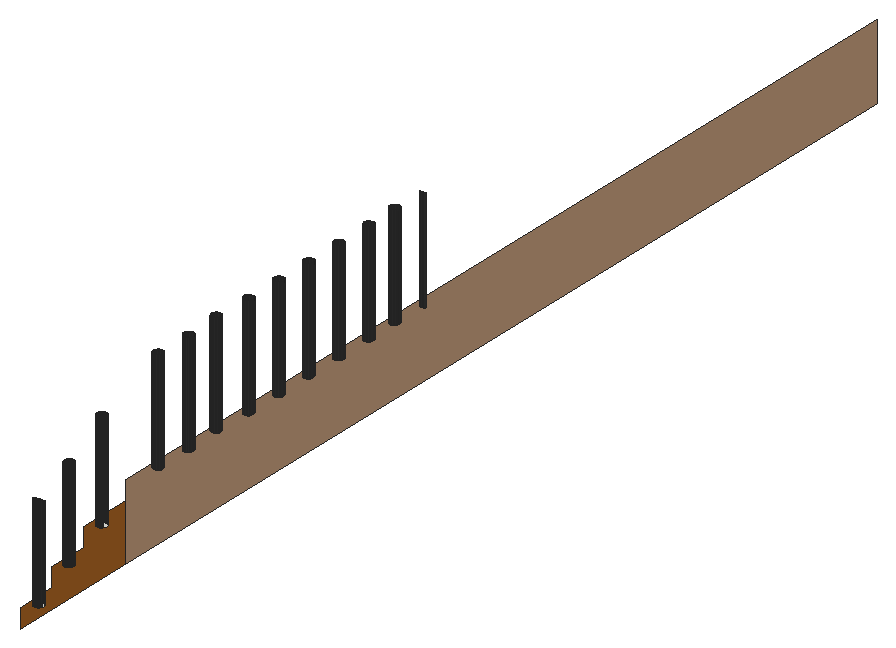
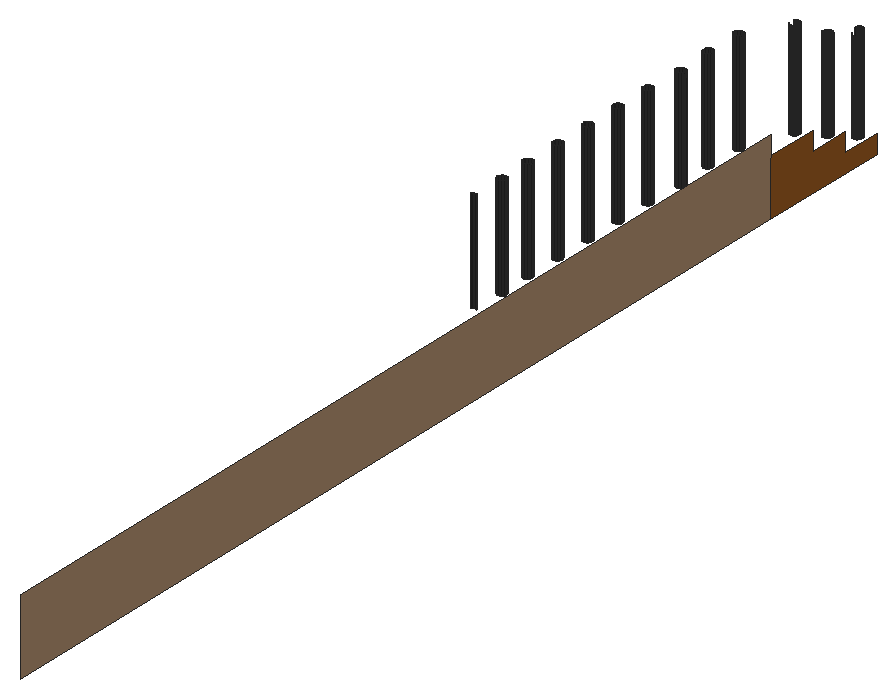
# SketchUp Ruby script. Lengths in inches.
U = 1.inch
M = Sketchup.active_model
def pt(a) = Geom::Point3d.new(a.map { |v| v * U })
def face(e, loops, mat)
  f = e.add_face(loops[0].map { |a| pt(a) })
  loops[1..].each { |l| e.add_face(l.map { |a| pt(a) }).erase! }
  f.material = f.back_material = mat if mat
  f
end
# faces: each face lists its corners as indices into pts; further lists are holes
def faces(e, pts, list, mat = nil) = list.each { |f| face(e, (f[0].is_a?(Array) ? f : [f]).map { |l| l.map { |i| pts[i] } }, mat) }
# xy, xz, yz: faces in a plane at the given z, y or x. An outline is a flat list of corners, or four numbers for a rectangle; further outlines are holes
def ring(l) = l.size == 4 ? [[l[0], l[1]], [l[2], l[1]], [l[2], l[3]], [l[0], l[3]]] : l.each_slice(2).to_a
def flat(e, list, mat, &to3) = list.each { |f| face(e, (f[0].is_a?(Array) ? f : [f]).map { |l| ring(l).map { |u, v| to3.(u, v) } }, mat) }
def xy(e, z, list, mat = nil) = flat(e, list, mat) { |x, y| [x, y, z] }
def xz(e, y, list, mat = nil) = flat(e, list, mat) { |x, z| [x, y, z] }
def yz(e, x, list, mat = nil) = flat(e, list, mat) { |y, z| [x, y, z] }
def lines(e, pts, list) = list.each { |a, b| e.add_line(pt(pts[a]), pt(pts[b])) }
# prism: a flat outline (further loops are holes) pulled along v
def prism(e, loops, v, mat = nil)
  f = face(e, loops, mat); d = Geom::Vector3d.new(v.map { |x| x * U })
  f.pushpull(f.normal.samedirection?(d) ? d.length : -d.length)
end
def box(e, o, s, mat = nil) = prism(e, [[o, [o[0] + s[0], o[1], o[2]], [o[0] + s[0], o[1] + s[1], o[2]], [o[0], o[1] + s[1], o[2]]]], [0, 0, s[2]], mat)
def at(x, y, z, deg = 0) = Geom::Transformation.translation(pt([x, y, z])) * Geom::Transformation.rotation(ORIGIN, Z_AXIS, deg.degrees)
def axes(o, x, y, z) = Geom::Transformation.new([*x, 0, *y, 0, *z, 0, *pt(o).to_a, 1])
def part(name) = M.definitions.add(name)
# library, detail: a bought-in or finely detailed component or shape, given as its bounding box
def library(name, o, s) = part(name).tap { |d| box(d.entities, o, s) }
def detail(e, o, s) = box(e.add_group.entities, o, s)
def put(e, d, t, mat = nil) = e.add_instance(d, t).tap { |i| i.material = mat if mat }
def group(e, t, mat = nil) = e.add_group.tap { |g| g.transformation = t; g.material = mat if mat }.entities
root = M.entities
M.materials.add("[0137_Black]").color = [45, 45, 45]
M.materials.add("[Stone Masonry Multi]").color = [182, 147, 116]
M.materials.add("[Wood Square Tile 02]").color = [160, 95, 34]
xy(root,12,[[5.2,5.16,4.89,5.1875,4.58,5.25,4.28,5.34,3.99,5.47,3.72,5.62,3.46,5.8,3.23,6.01,3.01,6.24,2.83,6.49,2.67,6.76,2.53,7.05,2.43,7.35,2.37,7.65,2.33,7.96,2.33,8.28,2.36,8.59,2.42,8.9,2.51,9.2,2.64,9.49,2.79,9.76,2.97,10.02,3.18,10.25,3.41,10.47,3.66,10.65,3.93,10.8125,4.22,10.94,4.52,11.04,4.82,11.11,5.13,11.15,5.45,11.15,5.76,11.12,6.07,11.0625,6.37,10.97,6.66,10.84,6.93,10.6875,7.1875,10.51,7.42,10.3,7.63,10.07,7.82,9.82,7.98,9.55,8.11,9.26,8.21,8.96,8.28,8.66,8.32,8.34,8.32,8.03,8.29,7.72,8.23,7.41,8.14,7.11,8.01,6.82,7.86,6.55,7.68,6.29,7.47,6.06,7.24,5.84,6.99,5.66,6.71,5.5,6.43,5.37,6.13,5.27,5.83,5.2,5.51,5.16]])
xy(root,24,[[4.7,30.03,4.39,30.06,4.08,30.12,3.78,30.22,3.49,30.34,3.22,30.49,2.96,30.68,2.73,30.88,2.51,31.11,2.33,31.37,2.17,31.64,2.04,31.92,1.9375,32.22,1.87,32.53,1.83,32.84,1.83,33.15,1.86,33.46,1.92,33.77,2.01,34.07,2.14,34.36,2.29,34.63,2.47,34.89,2.68,35.125,2.91,35.34,3.16,35.53,3.43,35.6875,3.72,35.82,4.02,35.92,4.32,35.99,4.63,36.02,4.95,36.03,5.26,36,5.57,35.93,5.87,35.84,6.16,35.72,6.43,35.5625,6.6875,35.38,6.92,35.17,7.14,34.94,7.32,34.6875,7.48,34.42,7.61,34.13,7.71,33.84,7.78,33.53,7.82,33.22,7.82,32.9,7.79,32.59,7.73,32.28,7.64,31.98,7.51,31.7,7.36,31.42,7.18,31.17,6.97,30.93,6.74,30.72,6.49,30.53,6.22,30.37,5.93,30.24,5.63,30.14,5.33,30.07,5.01,30.03]])
xy(root,36,[[5.56,55.09,5.25,55.12,4.94,55.18,4.64,55.27,4.35,55.4,4.08,55.55,3.82,55.74,3.59,55.94,3.375,56.17,3.1875,56.43,3.03,56.7,2.9,56.98,2.8,57.28,2.73,57.59,2.69,57.9,2.6875,58.21,2.72,58.52,2.78,58.83,2.87,59.13,3,59.42,3.15,59.69,3.33,59.95,3.54,60.19,3.77,60.4,4.02,60.59,4.29,60.75,4.58,60.875,4.875,60.98,5.18,61.05,5.49,61.08,5.81,61.08,6.12,61.06,6.43,60.99,6.73,60.9,7.02,60.78,7.29,60.62,7.55,60.4375,7.78,60.23,7.99,60,8.18,59.75,8.34,59.48,8.47,59.19,8.57,58.9,8.64,58.59,8.68,58.28,8.68,57.96,8.65,57.65,8.59,57.34,8.5,57.04,8.37,56.75,8.22,56.48,8.04,56.23,7.83,55.99,7.6,55.78,7.35,55.59,7.08,55.43,6.79,55.3,6.49,55.2,6.1875,55.13,5.875,55.09]])
xz(root,5.16,[[5.2,12,5.51,12,5.51,73.68,5.2,73.69]],"[0137_Black]")
xz(root,11.15,[[5.13,12,5.13,70.32,5.45,70.31,5.45,12]],"[0137_Black]")
xz(root,30.03,[[4.7,24,5.01,82.48]],"[0137_Black]")
xz(root,55.09,[[5.56,36,5.875,98.83]],"[0137_Black]")
xz(root,61.08,[[5.49,36,5.81,98.83]],"[0137_Black]")
yz(root,0,[[84,0,684,48]],"[Stone Masonry Multi]")
yz(root,0,[[0,0,0,12,25.4375,12,25.4375,24,50.75,24,50.75,36,84,36,84,0]],"[Wood Square Tile 02]")
yz(root,1.83,[[32.84,24,33.15,82.48]],"[0137_Black]")
yz(root,2.33,[[7.96,12,7.96,72.1,8.28,71.92,8.28,12]],"[0137_Black]")
yz(root,7.82,[[32.9,24,33.22,82.48]],"[0137_Black]")
p = [[4.28,5.34,12],[4.58,5.25,12],[4.58,5.25,73.63],[4.28,5.34,73.58],[4.89,5.1875,12],[4.89,5.1875,73.67],
  [5.2,5.16,12],[5.2,5.16,73.69],[5.51,5.16,12],[5.83,5.2,12],[5.83,5.2,73.66],[5.51,5.16,73.68],
  [6.13,5.27,12],[6.13,5.27,73.625],[3.99,5.47,12],[3.99,5.47,73.51],[6.43,5.37,12],[6.43,5.37,73.57],
  [6.71,5.5,12],[6.71,5.5,73.5],[3.72,5.62,12],[3.72,5.62,73.42],[6.99,5.66,12],[6.99,5.66,73.41],
  [3.46,5.8,12],[3.46,5.8,73.32],[7.24,5.84,12],[7.24,5.84,73.3],[3.23,6.01,12],[3.23,6.01,73.2],
  [7.47,6.06,12],[7.47,6.06,73.18],[3.01,6.24,12],[3.01,6.24,73.07],[7.68,6.29,12],[7.68,6.29,73.05],
  [2.83,6.49,12],[2.83,6.49,72.93],[7.86,6.55,12],[7.86,6.55,72.91],[2.67,6.76,12],[2.67,6.76,72.78],
  [8.01,6.82,12],[8.01,6.82,72.76],[2.53,7.05,12],[2.53,7.05,72.62],[2.43,7.35,12],[2.43,7.35,72.45],
  [2.37,7.65,12],[2.37,7.65,72.28],[2.33,7.96,12],[2.33,7.96,72.1],[2.36,8.59,12],[2.33,8.28,12],
  [2.33,8.28,71.92],[2.36,8.59,71.75],[2.42,8.9,12],[2.42,8.9,71.57],[2.51,9.2,12],[2.51,9.2,71.41],
  [2.64,9.49,12],[2.64,9.49,71.24],[2.79,9.76,12],[2.79,9.76,71.09],[7.98,9.55,12],[7.82,9.82,12],
  [7.82,9.82,71.07],[7.98,9.55,71.22],[2.97,10.02,12],[2.97,10.02,70.95],[7.63,10.07,12],[7.63,10.07,70.93],
  [3.18,10.25,12],[3.18,10.25,70.82],[7.42,10.3,12],[7.42,10.3,70.8],[3.41,10.47,12],[3.41,10.47,70.7],
  [7.1875,10.51,12],[7.1875,10.51,70.68],[3.66,10.65,12],[3.66,10.65,70.59],[6.93,10.6875,12],[6.93,10.6875,70.58],
  [3.93,10.8125,12],[3.93,10.8125,70.5],[6.66,10.84,12],[6.66,10.84,70.49],[4.22,10.94,12],[4.22,10.94,70.43],
  [6.37,10.97,12],[6.37,10.97,70.42],[4.52,11.04,12],[4.52,11.04,70.375],[4.82,11.11,12],[4.82,11.11,70.34],
  [6.07,11.0625,12],[6.07,11.0625,70.37],[5.13,11.15,12],[5.13,11.15,70.32],[5.76,11.12,12],[5.45,11.15,12],
  [5.45,11.15,70.31],[5.76,11.12,70.33],[4.39,30.06,24],[4.7,30.03,24],[4.7,30.03,82.48],[4.39,30.06,82.48],
  [5.01,30.03,24],[5.33,30.07,24],[5.33,30.07,82.48],[5.01,30.03,82.48],[3.78,30.22,24],[4.08,30.12,24],
  [4.08,30.12,82.48],[3.78,30.22,82.48],[5.63,30.14,24],[5.63,30.14,82.48],[5.93,30.24,24],[5.93,30.24,82.48],
  [3.49,30.34,24],[3.49,30.34,82.48],[6.22,30.37,24],[6.22,30.37,82.48],[3.22,30.49,24],[3.22,30.49,82.48],
  [6.49,30.53,24],[6.49,30.53,82.48],[2.96,30.68,24],[2.96,30.68,82.48],[6.74,30.72,24],[6.74,30.72,82.48],
  [2.73,30.88,24],[2.73,30.88,82.48],[6.97,30.93,24],[6.97,30.93,82.48],[2.51,31.11,24],[2.51,31.11,82.48],
  [7.18,31.17,24],[7.18,31.17,82.48],[2.33,31.37,24],[2.33,31.37,82.48],[7.36,31.42,24],[7.36,31.42,82.48],
  [2.17,31.64,24],[2.17,31.64,82.48],[7.51,31.7,24],[7.51,31.7,82.48],[2.04,31.92,24],[2.04,31.92,82.48],
  [7.64,31.98,24],[7.64,31.98,82.48],[1.9375,32.22,24],[1.9375,32.22,82.48],[7.73,32.28,24],[7.73,32.28,82.48],
  [1.87,32.53,24],[1.87,32.53,82.48],[7.79,32.59,24],[7.79,32.59,82.48],[1.83,32.84,24],[1.83,32.84,82.48],
  [7.82,32.9,24],[7.82,32.9,82.48],[1.86,33.46,24],[1.83,33.15,24],[1.83,33.15,82.48],[1.86,33.46,82.48],
  [7.82,33.22,24],[7.78,33.53,24],[7.78,33.53,82.48],[7.82,33.22,82.48],[1.92,33.77,24],[1.92,33.77,82.48],
  [7.71,33.84,24],[7.71,33.84,82.48],[2.01,34.07,24],[2.01,34.07,82.48],[7.61,34.13,24],[7.61,34.13,82.48],
  [2.14,34.36,24],[2.14,34.36,82.48],[7.48,34.42,24],[7.48,34.42,82.48],[2.29,34.63,24],[2.29,34.63,82.48],
  [7.32,34.6875,24],[7.32,34.6875,82.48],[2.47,34.89,24],[2.47,34.89,82.48],[7.14,34.94,24],[7.14,34.94,82.48],
  [2.68,35.125,24],[2.68,35.125,82.48],[6.92,35.17,24],[6.92,35.17,82.48],[2.91,35.34,24],[2.91,35.34,82.48],
  [6.6875,35.38,24],[6.6875,35.38,82.48],[3.16,35.53,24],[3.16,35.53,82.48],[6.43,35.5625,24],[6.43,35.5625,82.48],
  [3.43,35.6875,24],[3.43,35.6875,82.48],[6.16,35.72,24],[6.16,35.72,82.48],[3.72,35.82,24],[3.72,35.82,82.48],
  [5.87,35.84,24],[5.87,35.84,82.48],[4.02,35.92,24],[4.02,35.92,82.48],[5.57,35.93,24],[5.57,35.93,82.48],
  [4.32,35.99,24],[4.32,35.99,82.48],[5.26,36,24],[5.26,36,82.48],[4.63,36.02,24],[4.63,36.02,82.48],
  [4.95,36.03,24],[4.95,36.03,82.48],[4.94,55.18,36],[5.25,55.12,36],[5.25,55.12,98.83],[4.94,55.18,98.83],
  [5.56,55.09,36],[5.56,55.09,98.83],[5.875,55.09,36],[6.1875,55.13,36],[6.1875,55.13,97.28],[6.1875,55.13,98.83],
  [5.875,55.09,98.83],[6.49,55.2,36],[6.49,55.2,98.83],[4.64,55.27,36],[4.64,55.27,98.83],[4.64,55.27,97.19],
  [6.79,55.3,36],[6.79,55.3,98.83],[4.35,55.4,36],[4.35,55.4,98.83],[7.08,55.43,36],[7.08,55.43,98.83],
  [4.08,55.55,36],[4.08,55.55,98.83],[7.35,55.59,36],[7.35,55.59,98.83],[3.82,55.74,36],[3.82,55.74,98.83],
  [7.6,55.78,36],[7.6,55.78,98.83],[3.59,55.94,36],[3.59,55.94,98.83],[7.83,55.99,36],[7.83,55.99,98.83],
  [3.375,56.17,36],[3.375,56.17,98.83],[8.04,56.23,36],[8.04,56.23,98.83],[3.1875,56.43,36],[3.1875,56.43,98.83],
  [3.03,56.7,36],[3.03,56.7,98.83],[2.9,56.98,36],[2.9,56.98,98.83],[2.8,57.28,36],[2.8,57.28,98.83],
  [2.73,57.59,36],[2.73,57.59,98.83],[2.69,57.9,36],[2.69,57.9,98.83],[2.6875,58.21,36],[2.6875,58.21,98.83],
  [2.72,58.52,36],[2.72,58.52,98.83],[2.78,58.83,36],[2.78,58.83,98.83],[2.87,59.13,36],[2.87,59.13,98.83],
  [3,59.42,36],[3,59.42,98.83],[3.15,59.69,36],[3.15,59.69,98.83],[3.33,59.95,36],[3.33,59.95,98.83],
  [3.54,60.19,36],[3.54,60.19,98.83],[7.99,60,36],[7.78,60.23,36],[7.78,60.23,98.83],[7.99,60,98.83],
  [3.77,60.4,36],[3.77,60.4,98.83],[7.55,60.4375,36],[7.55,60.4375,98.83],[4.02,60.59,36],[4.02,60.59,98.83],
  [7.29,60.62,36],[7.29,60.62,98.83],[4.29,60.75,36],[4.29,60.75,98.83],[7.02,60.78,36],[7.02,60.78,98.83],
  [4.58,60.875,36],[4.58,60.875,98.83],[6.73,60.9,36],[6.73,60.9,98.83],[4.875,60.98,36],[4.875,60.98,98.83],
  [6.43,60.99,36],[6.43,60.99,98.83],[5.18,61.05,36],[5.18,61.05,98.83],[5.49,61.08,36],[5.49,61.08,98.83],
  [6.12,61.06,36],[6.12,61.06,98.83],[5.81,61.08,36],[5.81,61.08,98.83],[3.61,101.85,48],[4.38,101.75,48],
  [4.38,101.75,113.8],[3.61,101.85,113.8],[5,101.83,48],[5.16,101.85,48],[5.16,101.85,113.8],[2.88,102.15,48],
  [2.88,102.15,113.8],[5.88,102.15,48],[5.88,102.15,113.8],[2.26,102.625,48],[2.26,102.625,113.8],[6.5,102.625,48],
  [6.5,102.625,113.8],[1.78,103.25,48],[1.78,103.25,113.8],[6.98,103.25,48],[6.98,103.25,113.8],[1.48,103.97,48],
  [1.48,103.97,113.8],[7.28,103.97,48],[7.28,103.97,113.8],[1.38,104.75,48],[1.38,104.75,113.8],[7.38,104.75,48],
  [7.38,104.75,113.8],[1.48,105.52,48],[1.48,105.52,113.8],[7.28,105.52,48],[7.28,105.52,113.8],[1.78,106.25,48],
  [1.78,106.25,113.8],[6.98,106.25,48],[6.98,106.25,113.8],[2.26,106.87,48],[2.26,106.87,113.8],[6.5,106.87,48],
  [6.5,106.87,113.8],[2.88,107.34,48],[2.88,107.34,113.8],[5.88,107.34,48],[5.88,107.34,113.8],[3.61,107.64,48],
  [3.61,107.64,113.8],[5.16,107.64,48],[5.16,107.64,113.8],[4.38,107.75,48],[4.38,107.75,113.8],[5,107.66,48],
  [4.23,125.37,48],[5,125.27,48],[5,125.27,113.71],[5,125.27,113.8],[4.23,125.37,113.8],[4.23,125.37,113.61],
  [5.78,125.37,48],[5.78,125.37,113.8],[3.5,125.67,48],[3.5,125.67,113.8],[6.5,125.67,48],[6.5,125.67,113.8],
  [2.88,126.15,48],[2.88,126.15,113.8],[7.125,126.15,48],[7.125,126.15,113.8],[2.4,126.77,48],[2.4,126.77,113.8],
  [7.6,126.77,48],[7.6,126.77,113.8],[2.11,127.49,48],[2.11,127.49,113.8],[7.9,127.49,48],[7.9,127.49,113.8],
  [2,128.27,48],[2,128.27,113.8],[2.11,129.05,48],[2.11,129.05,113.8],[2.4,129.77,48],[2.4,129.77,113.8],
  [7.9,129.05,48],[7.6,129.77,48],[7.6,129.77,113.8],[7.9,129.05,113.8],[2.88,130.39,48],[2.88,130.39,113.8],
  [7.125,130.39,48],[7.125,130.39,113.8],[3.5,130.87,48],[3.5,130.87,113.8],[6.5,130.87,48],[6.5,130.87,113.8],
  [4.23,131.17,48],[4.23,131.17,113.8],[4.23,131.17,113.61],[5.78,131.17,48],[5.78,131.17,113.8],[5,131.27,48],
  [5,131.27,113.8],[5,131.27,113.71],[2.67,149.37,48],[3.45,149.27,48],[3.45,149.27,113.71],[3.45,149.27,113.8],
  [2.67,149.37,113.8],[4.23,149.37,48],[4.23,149.37,113.61],[4.23,149.37,113.8],[1.95,149.67,48],[1.95,149.67,113.8],
  [4.95,149.67,48],[4.95,149.67,113.8],[1.33,150.15,48],[1.33,150.15,113.8],[5,149.71,48],[5.57,150.15,48],
  [5.57,150.15,113.8],[0.85,150.77,48],[0.85,150.77,113.8],[6.05,150.77,48],[6.05,150.77,113.8],[0.55,151.49,48],
  [0.55,151.49,113.8],[6.35,151.49,48],[6.35,151.49,113.8],[0.45,152.27,48],[0.45,152.27,113.8],[6.45,152.27,48],
  [6.45,152.27,113.8],[0.55,153.05,48],[0.55,153.05,113.8],[6.35,153.05,48],[6.35,153.05,113.8],[0.85,153.77,48],
  [0.85,153.77,113.8],[6.05,153.77,48],[6.05,153.77,113.8],[1.33,154.39,48],[1.33,154.39,113.8],[5.57,154.39,48],
  [5.57,154.39,113.8],[1.95,154.87,48],[1.95,154.87,113.8],[5,154.83,48],[4.95,154.87,48],[4.95,154.87,113.8],
  [2.67,155.17,48],[2.67,155.17,113.8],[4.23,155.17,48],[4.23,155.17,113.61],[4.23,155.17,113.8],[3.45,155.27,48],
  [3.45,155.27,113.8],[3.45,155.27,113.71],[4.23,173.37,48],[5,173.27,48],[5,173.27,113.71],[5,173.27,113.8],
  [4.23,173.37,113.8],[4.23,173.37,113.61],[5.78,173.37,48],[5.78,173.37,113.8],[3.5,173.67,48],[3.5,173.67,113.8],
  [6.5,173.67,48],[6.5,173.67,113.8],[2.88,174.15,48],[2.88,174.15,113.8],[7.125,174.15,48],[7.125,174.15,113.8],
  [2.4,174.77,48],[2.4,174.77,113.8],[7.6,174.77,48],[7.6,174.77,113.8],[2.11,175.49,48],[2.11,175.49,113.8],
  [7.9,175.49,48],[7.9,175.49,113.8],[2,176.27,48],[2,176.27,113.8],[2.11,177.05,48],[2.11,177.05,113.8],
  [2.4,177.77,48],[2.4,177.77,113.8],[7.9,177.05,48],[7.6,177.77,48],[7.6,177.77,113.8],[7.9,177.05,113.8],
  [2.88,178.39,48],[2.88,178.39,113.8],[7.125,178.39,48],[7.125,178.39,113.8],[3.5,178.87,48],[3.5,178.87,113.8],
  [6.5,178.87,48],[6.5,178.87,113.8],[4.23,179.17,48],[4.23,179.17,113.8],[4.23,179.17,113.61],[5.78,179.17,48],
  [5.78,179.17,113.8],[5,179.27,48],[5,179.27,113.8],[5,179.27,113.71],[4.23,197.37,48],[5,197.27,48],
  [5,197.27,113.71],[5,197.27,113.8],[4.23,197.37,113.8],[4.23,197.37,113.61],[5.78,197.37,48],[5.78,197.37,113.8],
  [3.5,197.67,48],[3.5,197.67,113.8],[6.5,197.67,48],[6.5,197.67,113.8],[2.88,198.15,48],[2.88,198.15,113.8],
  [7.125,198.15,48],[7.125,198.15,113.8],[2.4,198.77,48],[2.4,198.77,113.8],[7.6,198.77,48],[7.6,198.77,113.8],
  [2.11,199.49,48],[2.11,199.49,113.8],[7.9,199.49,48],[7.9,199.49,113.8],[2,200.27,48],[2,200.27,113.8],
  [2.11,201.05,48],[2.11,201.05,113.8],[2.4,201.77,48],[2.4,201.77,113.8],[7.9,201.05,48],[7.6,201.77,48],
  [7.6,201.77,113.8],[7.9,201.05,113.8],[2.88,202.39,48],[2.88,202.39,113.8],[7.125,202.39,48],[7.125,202.39,113.8],
  [3.5,202.87,48],[3.5,202.87,113.8],[6.5,202.87,48],[6.5,202.87,113.8],[4.23,203.17,48],[4.23,203.17,113.8],
  [4.23,203.17,113.61],[5.78,203.17,48],[5.78,203.17,113.8],[5,203.27,48],[5,203.27,113.8],[5,203.27,113.71],
  [4.23,221.37,48],[5,221.27,48],[5,221.27,113.71],[5,221.27,113.8],[4.23,221.37,113.8],[4.23,221.37,113.61],
  [5.78,221.37,48],[5.78,221.37,113.8],[3.5,221.67,48],[3.5,221.67,113.8],[6.5,221.67,48],[6.5,221.67,113.8],
  [2.88,222.15,48],[2.88,222.15,113.8],[7.125,222.15,48],[7.125,222.15,113.8],[2.4,222.77,48],[2.4,222.77,113.8],
  [7.6,222.77,48],[7.6,222.77,113.8],[2.11,223.49,48],[2.11,223.49,113.8],[7.9,223.49,48],[7.9,223.49,113.8],
  [2,224.27,48],[2,224.27,113.8],[2.11,225.05,48],[2.11,225.05,113.8],[2.4,225.77,48],[2.4,225.77,113.8],
  [7.9,225.05,48],[7.6,225.77,48],[7.6,225.77,113.8],[7.9,225.05,113.8],[2.88,226.39,48],[2.88,226.39,113.8],
  [7.125,226.39,48],[7.125,226.39,113.8],[3.5,226.87,48],[3.5,226.87,113.8],[6.5,226.87,48],[6.5,226.87,113.8],
  [4.23,227.17,48],[4.23,227.17,113.8],[4.23,227.17,113.61],[5.78,227.17,48],[5.78,227.17,113.8],[5,227.27,48],
  [5,227.27,113.8],[5,227.27,113.71],[4.23,245.37,48],[5,245.27,48],[5,245.27,113.71],[5,245.27,113.8],
  [4.23,245.37,113.8],[4.23,245.37,113.61],[5.78,245.37,48],[5.78,245.37,113.8],[3.5,245.67,48],[3.5,245.67,113.8],
  [6.5,245.67,48],[6.5,245.67,113.8],[2.88,246.15,48],[2.88,246.15,113.8],[7.125,246.15,48],[7.125,246.15,113.8],
  [2.4,246.77,48],[2.4,246.77,113.8],[7.6,246.77,48],[7.6,246.77,113.8],[2.11,247.49,48],[2.11,247.49,113.8],
  [7.9,247.49,48],[7.9,247.49,113.8],[2,248.27,48],[2,248.27,113.8],[2.11,249.05,48],[2.11,249.05,113.8],
  [2.4,249.77,48],[2.4,249.77,113.8],[7.9,249.05,48],[7.6,249.77,48],[7.6,249.77,113.8],[7.9,249.05,113.8],
  [2.88,250.39,48],[2.88,250.39,113.8],[7.125,250.39,48],[7.125,250.39,113.8],[3.5,250.87,48],[3.5,250.87,113.8],
  [6.5,250.87,48],[6.5,250.87,113.8],[4.23,251.17,48],[4.23,251.17,113.8],[4.23,251.17,113.61],[5.78,251.17,48],
  [5.78,251.17,113.8],[5,251.27,48],[5,251.27,113.8],[5,251.27,113.71],[4.23,269.37,48],[5,269.27,48],
  [5,269.27,113.71],[5,269.27,113.8],[4.23,269.37,113.8],[4.23,269.37,113.61],[5.78,269.37,48],[5.78,269.37,113.8],
  [3.5,269.67,48],[3.5,269.67,113.8],[6.5,269.67,48],[6.5,269.67,113.8],[2.88,270.15,48],[2.88,270.15,113.8],
  [7.125,270.15,48],[7.125,270.15,113.8],[2.4,270.77,48],[2.4,270.77,113.8],[7.6,270.77,48],[7.6,270.77,113.8],
  [2.11,271.49,48],[2.11,271.49,113.8],[7.9,271.49,48],[7.9,271.49,113.8],[2,272.27,48],[2,272.27,113.8],
  [2.11,273.05,48],[2.11,273.05,113.8],[2.4,273.77,48],[2.4,273.77,113.8],[7.9,273.05,48],[7.6,273.77,48],
  [7.6,273.77,113.8],[7.9,273.05,113.8],[2.88,274.39,48],[2.88,274.39,113.8],[7.125,274.39,48],[7.125,274.39,113.8],
  [3.5,274.87,48],[3.5,274.87,113.8],[6.5,274.87,48],[6.5,274.87,113.8],[4.23,275.17,48],[4.23,275.17,113.8],
  [4.23,275.17,113.61],[5.78,275.17,48],[5.78,275.17,113.8],[5,275.27,48],[5,275.27,113.8],[5,275.27,113.71],
  [3.61,290.74,48],[4.38,290.63,48],[4.38,290.63,113.8],[3.61,290.74,113.8],[5,290.72,48],[5.16,290.74,48],
  [5.16,290.74,113.8],[2.88,291.04,48],[2.88,291.04,113.8],[5.88,291.04,48],[5.88,291.04,113.8],[2.26,291.51,48],
  [2.26,291.51,113.8],[6.5,291.51,48],[6.5,291.51,113.8],[1.78,292.13,48],[1.78,292.13,113.8],[6.98,292.13,48],
  [6.98,292.13,113.8],[1.48,292.86,48],[1.48,292.86,113.8],[7.28,292.86,48],[7.28,292.86,113.8],[1.38,293.63,48],
  [1.38,293.63,113.8],[7.38,293.63,48],[7.38,293.63,113.8],[1.48,294.41,48],[1.48,294.41,113.8],[7.28,294.41,48],
  [7.28,294.41,113.8],[1.78,295.13,48],[1.78,295.13,113.8],[6.98,295.13,48],[6.98,295.13,113.8],[2.26,295.76,48],
  [2.26,295.76,113.8],[6.5,295.76,48],[6.5,295.76,113.8],[2.88,296.23,48],[2.88,296.23,113.8],[5.88,296.23,48],
  [5.88,296.23,113.8],[3.61,296.53,48],[3.61,296.53,113.8],[5.16,296.53,48],[5.16,296.53,113.8],[4.38,296.63,48],
  [4.38,296.63,113.8],[5,296.55,48],[4.23,314.26,48],[5,314.16,48],[5,314.16,113.71],[5,314.16,113.8],
  [4.23,314.26,113.8],[4.23,314.26,113.61],[5.78,314.26,48],[5.78,314.26,113.8],[3.5,314.56,48],[3.5,314.56,113.8],
  [6.5,314.56,48],[6.5,314.56,113.8],[7.125,315.04,48],[7.125,315.04,113.8],[5.32,8.15,12],[5.32,8.15,72],
  [5.68,58.09,36],[5.68,58.09,98.83],[4.82,33.03,24],[4.82,33.03,82.48]]
faces(root,p,[[0,1,2,3],[1,4,5,2],[4,6,7,5],[8,9,10,11],[9,12,13,10],[14,0,3,15],[12,16,17,13],[16,18,19,17],
  [20,14,15,21],[18,22,23,19],[24,20,21,25],[22,26,27,23],[28,24,25,29],[26,30,31,27],[32,28,29,33],[30,34,35,31],
  [36,32,33,37],[34,38,39,35],[40,36,37,41],[38,42,43,39],[44,40,41,45],[46,44,45,47],[48,46,47,49],[50,48,49,51],
  [52,53,54,55],[56,52,55,57],[58,56,57,59],[60,58,59,61],[62,60,61,63],[64,65,66,67],[68,62,63,69],[65,70,71,66],
  [72,68,69,73],[70,74,75,71],[76,72,73,77],[74,78,79,75],[80,76,77,81],[78,82,83,79],[84,80,81,85],[82,86,87,83],
  [88,84,85,89],[86,90,91,87],[92,88,89,93],[94,92,93,95],[90,96,97,91],[98,94,95,99],[100,101,102,103],[96,100,103,97],
  [104,105,106,107],[108,109,110,111],[112,113,114,115],[113,104,107,114],[109,116,117,110],[116,118,119,117],[120,112,115,121],[118,122,123,119],
  [124,120,121,125],[122,126,127,123],[128,124,125,129],[126,130,131,127],[132,128,129,133],[130,134,135,131],[136,132,133,137],[134,138,139,135],
  [140,136,137,141],[138,142,143,139],[144,140,141,145],[142,146,147,143],[148,144,145,149],[146,150,151,147],[152,148,149,153],[150,154,155,151],
  [156,152,153,157],[154,158,159,155],[160,156,157,161],[158,162,163,159],[164,165,166,167],[168,169,170,171],[172,164,167,173],[169,174,175,170],
  [176,172,173,177],[174,178,179,175],[180,176,177,181],[178,182,183,179],[184,180,181,185],[182,186,187,183],[188,184,185,189],[186,190,191,187],
  [192,188,189,193],[190,194,195,191],[196,192,193,197],[194,198,199,195],[200,196,197,201],[198,202,203,199],[204,200,201,205],[202,206,207,203],
  [208,204,205,209],[206,210,211,207],[212,208,209,213],[210,214,215,211],[216,212,213,217],[214,218,219,215],[220,216,217,221],[222,220,221,223],
  [218,222,223,219],[224,225,226,227],[225,228,229,226],[230,231,232,233,234],[231,235,236,233,232],[237,224,227,238,239],[235,240,241,236],[242,237,239,238,243],
  [240,244,245,241],[246,242,243,247],[244,248,249,245],[250,246,247,251],[248,252,253,249],[254,250,251,255],[252,256,257,253],[258,254,255,259],
  [256,260,261,257],[262,258,259,263],[264,262,263,265],[266,264,265,267],[268,266,267,269],[270,268,269,271],[272,270,271,273],[274,272,273,275],
  [276,274,275,277],[278,276,277,279],[280,278,279,281],[282,280,281,283],[284,282,283,285],[286,284,285,287],[288,286,287,289],[290,291,292,293],
  [294,288,289,295],[291,296,297,292],[298,294,295,299],[296,300,301,297],[302,298,299,303],[300,304,305,301],[306,302,303,307],[304,308,309,305],
  [310,306,307,311],[308,312,313,309],[314,310,311,315],[316,314,315,317],[312,318,319,313],[318,320,321,319],[322,323,324,325],[323,326,327,328,324],
  [329,322,325,330],[327,331,332,328],[333,329,330,334],[331,335,336,332],[337,333,334,338],[335,339,340,336],[341,337,338,342],[339,343,344,340],
  [345,341,342,346],[343,347,348,344],[349,345,346,350],[347,351,352,348],[353,349,350,354],[351,355,356,352],[357,353,354,358],[355,359,360,356],
  [361,357,358,362],[359,363,364,360],[365,361,362,366],[363,367,368,364],[369,365,366,370],[367,371,369,370,368],[372,373,374,375,376,377],[373,378,379,375,374],
  [380,372,377,376,381],[378,382,383,379],[384,380,381,385],[382,386,387,383],[388,384,385,389],[386,390,391,387],[392,388,389,393],[390,394,395,391],
  [396,392,393,397],[398,396,397,399],[400,398,399,401],[402,403,404,405],[406,400,401,407],[403,408,409,404],[410,406,407,411],[408,412,413,409],
  [414,410,411,415,416],[412,417,418,413],[419,414,416,415,420,421],[417,419,421,420,418],[422,423,424,425,426],[423,427,428,429,425,424],[430,422,426,431],[427,432,433,429,428],
  [434,430,431,435],[432,436,437,438,433],[439,434,435,440],[437,441,442,438],[443,439,440,444],[441,445,446,442],[447,443,444,448],[445,449,450,446],
  [451,447,448,452],[449,453,454,450],[455,451,452,456],[453,457,458,454],[459,455,456,460],[457,461,462,458],[463,459,460,464],[461,465,466,467,462],
  [468,463,464,469],[466,470,471,472,467],[473,468,469,474,475],[470,473,475,474,472,471],[476,477,478,479,480,481],[477,482,483,479,478],[484,476,481,480,485],[482,486,487,483],
  [488,484,485,489],[486,490,491,487],[492,488,489,493],[490,494,495,491],[496,492,493,497],[494,498,499,495],[500,496,497,501],[502,500,501,503],
  [504,502,503,505],[506,507,508,509],[510,504,505,511],[507,512,513,508],[514,510,511,515],[512,516,517,513],[518,514,515,519,520],[516,521,522,517],
  [523,518,520,519,524,525],[521,523,525,524,522],[526,527,528,529,530,531],[527,532,533,529,528],[534,526,531,530,535],[532,536,537,533],[538,534,535,539],[536,540,541,537],
  [542,538,539,543],[540,544,545,541],[546,542,543,547],[544,548,549,545],[550,546,547,551],[552,550,551,553],[554,552,553,555],[556,557,558,559],
  [560,554,555,561],[557,562,563,558],[564,560,561,565],[562,566,567,563],[568,564,565,569,570],[566,571,572,567],[573,568,570,569,574,575],[571,573,575,574,572],
  [576,577,578,579,580,581],[577,582,583,579,578],[584,576,581,580,585],[582,586,587,583],[588,584,585,589],[586,590,591,587],[592,588,589,593],[590,594,595,591],
  [596,592,593,597],[594,598,599,595],[600,596,597,601],[602,600,601,603],[604,602,603,605],[606,607,608,609],[610,604,605,611],[607,612,613,608],
  [614,610,611,615],[612,616,617,613],[618,614,615,619,620],[616,621,622,617],[623,618,620,619,624,625],[621,623,625,624,622],[626,627,628,629,630,631],[627,632,633,629,628],
  [634,626,631,630,635],[632,636,637,633],[638,634,635,639],[636,640,641,637],[642,638,639,643],[640,644,645,641],[646,642,643,647],[644,648,649,645],
  [650,646,647,651],[652,650,651,653],[654,652,653,655],[656,657,658,659],[660,654,655,661],[657,662,663,658],[664,660,661,665],[662,666,667,663],
  [668,664,665,669,670],[666,671,672,667],[673,668,670,669,674,675],[671,673,675,674,672],[676,677,678,679,680,681],[677,682,683,679,678],[684,676,681,680,685],[682,686,687,683],
  [688,684,685,689],[686,690,691,687],[692,688,689,693],[690,694,695,691],[696,692,693,697],[694,698,699,695],[700,696,697,701],[702,700,701,703],
  [704,702,703,705],[706,707,708,709],[710,704,705,711],[707,712,713,708],[714,710,711,715],[712,716,717,713],[718,714,715,719,720],[716,721,722,717],
  [723,718,720,719,724,725],[721,723,725,724,722],[726,727,728,729],[727,730,731,732,728],[733,726,729,734],[731,735,736,732],[737,733,734,738],[735,739,740,736],
  [741,737,738,742],[739,743,744,740],[745,741,742,746],[743,747,748,744],[749,745,746,750],[747,751,752,748],[753,749,750,754],[751,755,756,752],
  [757,753,754,758],[755,759,760,756],[761,757,758,762],[759,763,764,760],[765,761,762,766],[763,767,768,764],[769,765,766,770],[767,771,772,768],
  [773,769,770,774],[771,775,773,774,772],[776,777,778,779,780,781],[777,782,783,779,778],[784,776,781,780,785],[782,786,787,783],[786,788,789,787]],"[0137_Black]")
lines(root,p,[[790,791],[792,793],[794,795]])
